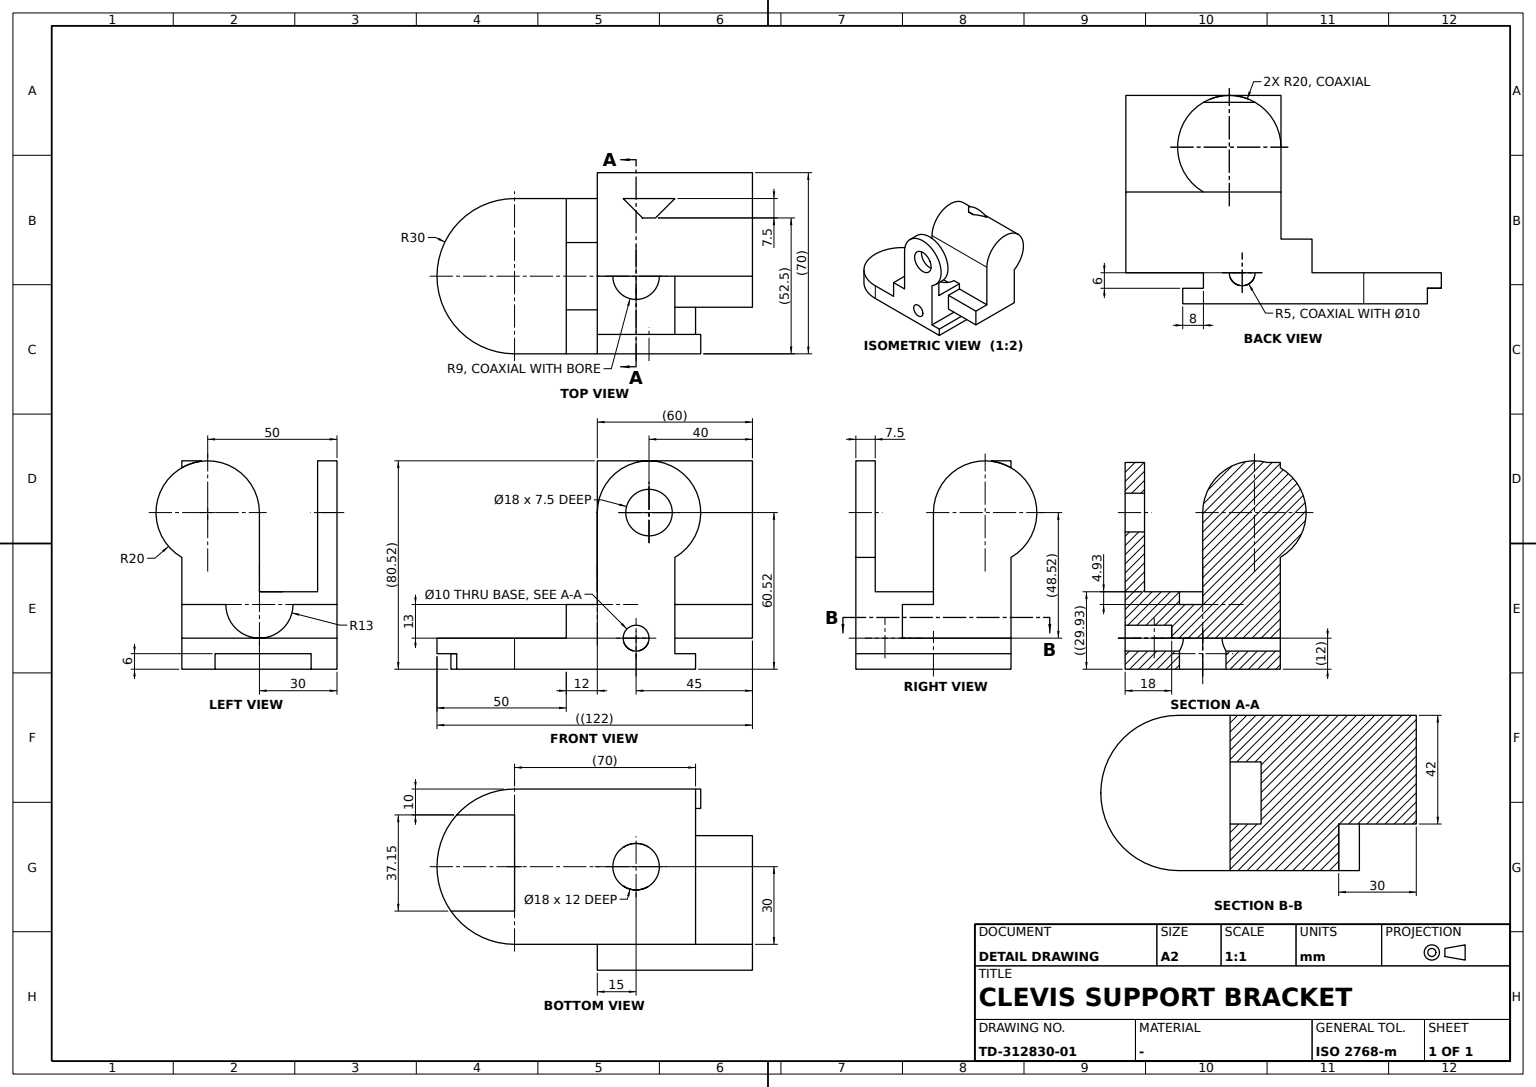
ISO-10303-21;
HEADER;
FILE_DESCRIPTION((''),'2;1');
FILE_NAME('','',(''),(''),'','','');
FILE_SCHEMA(('AUTOMOTIVE_DESIGN'));
ENDSEC;
DATA;
#1=APPLICATION_CONTEXT('');
#2=PRODUCT_CONTEXT('',#1,'mechanical');
#3=PRODUCT('','','',(#2));
#4=PRODUCT_DEFINITION_FORMATION('','',#3);
#5=PRODUCT_DEFINITION_CONTEXT('',#1,'design');
#6=PRODUCT_DEFINITION('','',#4,#5);
#7=PRODUCT_DEFINITION_SHAPE('','',#6);
#8=(LENGTH_UNIT()NAMED_UNIT(*)SI_UNIT(.MILLI.,.METRE.));
#9=(NAMED_UNIT(*)PLANE_ANGLE_UNIT()SI_UNIT($,.RADIAN.));
#10=(NAMED_UNIT(*)SI_UNIT($,.STERADIAN.)SOLID_ANGLE_UNIT());
#11=UNCERTAINTY_MEASURE_WITH_UNIT(LENGTH_MEASURE(1.E-05),#8,'distance_accuracy_value','');
#12=(GEOMETRIC_REPRESENTATION_CONTEXT(3)GLOBAL_UNCERTAINTY_ASSIGNED_CONTEXT((#11))GLOBAL_UNIT_ASSIGNED_CONTEXT((#8,#9,#10))REPRESENTATION_CONTEXT('',''));
#13=CARTESIAN_POINT('',(0.,-56.,25.));
#14=VERTEX_POINT('',#13);
#15=CARTESIAN_POINT('',(-9.,-47.,25.));
#16=VERTEX_POINT('',#15);
#17=CARTESIAN_POINT('',(0.,-47.,25.));
#18=DIRECTION('',(0.,0.,-1.));
#19=DIRECTION('',(0.,-1.,0.));
#20=AXIS2_PLACEMENT_3D('',#17,#18,#19);
#21=CIRCLE('',#20,9.);
#22=EDGE_CURVE('',#14,#16,#21,.T.);
#23=ORIENTED_EDGE('',*,*,#22,.F.);
#24=CARTESIAN_POINT('',(0.,-38.,25.));
#25=VERTEX_POINT('',#24);
#26=VECTOR('',#19,1000.);
#27=LINE('',#17,#26);
#28=EDGE_CURVE('',#25,#14,#27,.T.);
#29=ORIENTED_EDGE('',*,*,#28,.F.);
#30=EDGE_CURVE('',#16,#25,#21,.T.);
#31=ORIENTED_EDGE('',*,*,#30,.F.);
#32=EDGE_LOOP('',(#23,#29,#31));
#33=FACE_OUTER_BOUND('',#32,.T.);
#34=CARTESIAN_POINT('',(30.,-20.,25.));
#35=AXIS2_PLACEMENT_3D('',#34,#18,#19);
#36=PLANE('',#35);
#37=ADVANCED_FACE('',(#33),#36,.F.);
#38=CARTESIAN_POINT('',(-30.,0.,0.));
#39=VERTEX_POINT('',#38);
#40=CARTESIAN_POINT('',(-30.,0.,12.));
#41=VERTEX_POINT('',#40);
#42=CARTESIAN_POINT('',(-30.,0.,6.));
#43=DIRECTION('',(0.,0.,1.));
#44=VECTOR('',#43,1000.);
#45=LINE('',#42,#44);
#46=EDGE_CURVE('',#39,#41,#45,.T.);
#47=ORIENTED_EDGE('',*,*,#46,.F.);
#48=CARTESIAN_POINT('',(-30.,-20.,0.));
#49=VERTEX_POINT('',#48);
#50=CARTESIAN_POINT('',(-30.,-10.,0.));
#51=LINE('',#50,#26);
#52=EDGE_CURVE('',#39,#49,#51,.T.);
#53=ORIENTED_EDGE('',*,*,#52,.T.);
#54=CARTESIAN_POINT('',(-30.,-20.,12.));
#55=VERTEX_POINT('',#54);
#56=CARTESIAN_POINT('',(-30.,-20.,6.));
#57=LINE('',#56,#44);
#58=EDGE_CURVE('',#49,#55,#57,.T.);
#59=ORIENTED_EDGE('',*,*,#58,.T.);
#60=CARTESIAN_POINT('',(-30.,-10.,12.));
#61=LINE('',#60,#26);
#62=EDGE_CURVE('',#41,#55,#61,.T.);
#63=ORIENTED_EDGE('',*,*,#62,.F.);
#64=EDGE_LOOP('',(#47,#53,#59,#63));
#65=FACE_OUTER_BOUND('',#64,.T.);
#66=DIRECTION('',(-1.,0.,0.));
#67=AXIS2_PLACEMENT_3D('',#38,#66,#19);
#68=PLANE('',#67);
#69=ADVANCED_FACE('',(#65),#68,.T.);
#70=CARTESIAN_POINT('',(-12.,-92.,25.));
#71=VERTEX_POINT('',#70);
#72=CARTESIAN_POINT('',(0.,-92.,25.));
#73=VERTEX_POINT('',#72);
#74=CARTESIAN_POINT('',(-6.,-92.,25.));
#75=DIRECTION('',(1.,0.,0.));
#76=VECTOR('',#75,1000.);
#77=LINE('',#74,#76);
#78=EDGE_CURVE('',#71,#73,#77,.T.);
#79=ORIENTED_EDGE('',*,*,#78,.F.);
#80=CARTESIAN_POINT('',(-12.,-92.,12.));
#81=VERTEX_POINT('',#80);
#82=CARTESIAN_POINT('',(-12.,-92.,18.5));
#83=LINE('',#82,#44);
#84=EDGE_CURVE('',#81,#71,#83,.T.);
#85=ORIENTED_EDGE('',*,*,#84,.F.);
#86=CARTESIAN_POINT('',(30.,-92.,12.));
#87=VERTEX_POINT('',#86);
#88=CARTESIAN_POINT('',(9.,-92.,12.));
#89=VECTOR('',#66,1000.);
#90=LINE('',#88,#89);
#91=EDGE_CURVE('',#87,#81,#90,.T.);
#92=ORIENTED_EDGE('',*,*,#91,.F.);
#93=CARTESIAN_POINT('',(30.,-92.,43.201274));
#94=VERTEX_POINT('',#93);
#95=CARTESIAN_POINT('',(30.,-92.,27.600637));
#96=VECTOR('',#18,1000.);
#97=LINE('',#95,#96);
#98=EDGE_CURVE('',#94,#87,#97,.T.);
#99=ORIENTED_EDGE('',*,*,#98,.F.);
#100=CARTESIAN_POINT('',(0.,-92.,60.521782));
#101=VERTEX_POINT('',#100);
#102=CARTESIAN_POINT('',(20.,-92.,60.521782));
#103=DIRECTION('',(0.,1.,0.));
#104=AXIS2_PLACEMENT_3D('',#102,#103,#66);
#105=CIRCLE('',#104,20.);
#106=EDGE_CURVE('',#101,#94,#105,.T.);
#107=ORIENTED_EDGE('',*,*,#106,.F.);
#108=CARTESIAN_POINT('',(0.,-92.,42.760891));
#109=LINE('',#108,#44);
#110=EDGE_CURVE('',#73,#101,#109,.T.);
#111=ORIENTED_EDGE('',*,*,#110,.F.);
#112=EDGE_LOOP('',(#79,#85,#92,#99,#107,#111));
#113=FACE_OUTER_BOUND('',#112,.T.);
#114=CARTESIAN_POINT('',(0.,-92.,0.));
#115=AXIS2_PLACEMENT_3D('',#114,#103,#66);
#116=PLANE('',#115);
#117=ADVANCED_FACE('',(#113),#116,.F.);
#118=CARTESIAN_POINT('',(-9.,-47.,29.92601));
#119=VERTEX_POINT('',#118);
#120=CARTESIAN_POINT('',(-9.,-47.,14.303005));
#121=LINE('',#120,#96);
#122=EDGE_CURVE('',#119,#16,#121,.T.);
#123=ORIENTED_EDGE('',*,*,#122,.F.);
#124=CARTESIAN_POINT('',(0.,-56.,29.92601));
#125=VERTEX_POINT('',#124);
#126=CARTESIAN_POINT('',(0.,-47.,29.92601));
#127=AXIS2_PLACEMENT_3D('',#126,#18,#75);
#128=CIRCLE('',#127,9.);
#129=EDGE_CURVE('',#125,#119,#128,.T.);
#130=ORIENTED_EDGE('',*,*,#129,.F.);
#131=CARTESIAN_POINT('',(0.,-56.,27.463005));
#132=LINE('',#131,#96);
#133=EDGE_CURVE('',#125,#14,#132,.T.);
#134=ORIENTED_EDGE('',*,*,#133,.T.);
#135=ORIENTED_EDGE('',*,*,#22,.T.);
#136=EDGE_LOOP('',(#123,#130,#134,#135));
#137=FACE_OUTER_BOUND('',#136,.T.);
#138=CARTESIAN_POINT('',(0.,-47.,14.303005));
#139=AXIS2_PLACEMENT_3D('',#138,#43,#75);
#140=CYLINDRICAL_SURFACE('',#139,9.);
#141=ADVANCED_FACE('',(#137),#140,.F.);
#142=CARTESIAN_POINT('',(30.,-20.,12.));
#143=VERTEX_POINT('',#142);
#144=CARTESIAN_POINT('',(0.,-20.,12.));
#145=VERTEX_POINT('',#144);
#146=CARTESIAN_POINT('',(15.,-20.,12.));
#147=LINE('',#146,#89);
#148=EDGE_CURVE('',#143,#145,#147,.T.);
#149=ORIENTED_EDGE('',*,*,#148,.T.);
#150=CARTESIAN_POINT('',(13.,-20.,25.));
#151=VERTEX_POINT('',#150);
#152=CARTESIAN_POINT('',(0.,-20.,25.));
#153=AXIS2_PLACEMENT_3D('',#152,#103,#66);
#154=CIRCLE('',#153,13.);
#155=EDGE_CURVE('',#151,#145,#154,.T.);
#156=ORIENTED_EDGE('',*,*,#155,.F.);
#157=VERTEX_POINT('',#34);
#158=CARTESIAN_POINT('',(21.5,-20.,25.));
#159=LINE('',#158,#89);
#160=EDGE_CURVE('',#157,#151,#159,.T.);
#161=ORIENTED_EDGE('',*,*,#160,.F.);
#162=CARTESIAN_POINT('',(30.,-20.,18.5));
#163=LINE('',#162,#44);
#164=EDGE_CURVE('',#143,#157,#163,.T.);
#165=ORIENTED_EDGE('',*,*,#164,.F.);
#166=EDGE_LOOP('',(#149,#156,#161,#165));
#167=FACE_OUTER_BOUND('',#166,.T.);
#168=AXIS2_PLACEMENT_3D('',#142,#19,#43);
#169=PLANE('',#168);
#170=ADVANCED_FACE('',(#167),#169,.F.);
#171=CARTESIAN_POINT('',(30.,-70.,6.));
#172=VERTEX_POINT('',#171);
#173=CARTESIAN_POINT('',(30.,-62.,6.));
#174=VERTEX_POINT('',#173);
#175=CARTESIAN_POINT('',(30.,-66.,6.));
#176=VECTOR('',#103,1000.);
#177=LINE('',#175,#176);
#178=EDGE_CURVE('',#172,#174,#177,.T.);
#179=ORIENTED_EDGE('',*,*,#178,.T.);
#180=CARTESIAN_POINT('',(-30.,-62.,6.));
#181=VERTEX_POINT('',#180);
#182=CARTESIAN_POINT('',(0.,-62.,6.));
#183=LINE('',#182,#89);
#184=EDGE_CURVE('',#174,#181,#183,.T.);
#185=ORIENTED_EDGE('',*,*,#184,.T.);
#186=CARTESIAN_POINT('',(-30.,-70.,6.));
#187=VERTEX_POINT('',#186);
#188=CARTESIAN_POINT('',(-30.,-66.,6.));
#189=LINE('',#188,#176);
#190=EDGE_CURVE('',#187,#181,#189,.T.);
#191=ORIENTED_EDGE('',*,*,#190,.F.);
#192=CARTESIAN_POINT('',(0.,-70.,6.));
#193=LINE('',#192,#89);
#194=EDGE_CURVE('',#172,#187,#193,.T.);
#195=ORIENTED_EDGE('',*,*,#194,.F.);
#196=EDGE_LOOP('',(#179,#185,#191,#195));
#197=FACE_OUTER_BOUND('',#196,.T.);
#198=AXIS2_PLACEMENT_3D('',#173,#18,#19);
#199=PLANE('',#198);
#200=ADVANCED_FACE('',(#197),#199,.F.);
#201=CARTESIAN_POINT('',(0.,-38.,29.92601));
#202=VERTEX_POINT('',#201);
#203=EDGE_CURVE('',#119,#202,#128,.T.);
#204=ORIENTED_EDGE('',*,*,#203,.F.);
#205=ORIENTED_EDGE('',*,*,#122,.T.);
#206=ORIENTED_EDGE('',*,*,#30,.T.);
#207=CARTESIAN_POINT('',(0.,-38.,27.463005));
#208=LINE('',#207,#96);
#209=EDGE_CURVE('',#202,#25,#208,.T.);
#210=ORIENTED_EDGE('',*,*,#209,.F.);
#211=EDGE_LOOP('',(#204,#205,#206,#210));
#212=FACE_OUTER_BOUND('',#211,.T.);
#213=ADVANCED_FACE('',(#212),#140,.F.);
#214=CARTESIAN_POINT('',(30.,-70.,0.));
#215=VERTEX_POINT('',#214);
#216=CARTESIAN_POINT('',(30.,-70.,3.));
#217=LINE('',#216,#44);
#218=EDGE_CURVE('',#215,#172,#217,.T.);
#219=ORIENTED_EDGE('',*,*,#218,.T.);
#220=ORIENTED_EDGE('',*,*,#194,.T.);
#221=CARTESIAN_POINT('',(-30.,-70.,0.));
#222=VERTEX_POINT('',#221);
#223=CARTESIAN_POINT('',(-30.,-70.,3.));
#224=LINE('',#223,#44);
#225=EDGE_CURVE('',#222,#187,#224,.T.);
#226=ORIENTED_EDGE('',*,*,#225,.F.);
#227=CARTESIAN_POINT('',(0.,-70.,0.));
#228=LINE('',#227,#76);
#229=EDGE_CURVE('',#222,#215,#228,.T.);
#230=ORIENTED_EDGE('',*,*,#229,.T.);
#231=EDGE_LOOP('',(#219,#220,#226,#230));
#232=FACE_OUTER_BOUND('',#231,.T.);
#233=AXIS2_PLACEMENT_3D('',#221,#19,#75);
#234=PLANE('',#233);
#235=ADVANCED_FACE('',(#232),#234,.T.);
#236=CARTESIAN_POINT('',(-20.,0.,6.));
#237=VERTEX_POINT('',#236);
#238=CARTESIAN_POINT('',(17.153702,0.,6.));
#239=VERTEX_POINT('',#238);
#240=CARTESIAN_POINT('',(-1.423149,0.,6.));
#241=LINE('',#240,#76);
#242=EDGE_CURVE('',#237,#239,#241,.T.);
#243=ORIENTED_EDGE('',*,*,#242,.F.);
#244=CARTESIAN_POINT('',(-20.,22.36068,6.));
#245=VERTEX_POINT('',#244);
#246=CARTESIAN_POINT('',(-20.,11.18034,6.));
#247=LINE('',#246,#176);
#248=EDGE_CURVE('',#237,#245,#247,.T.);
#249=ORIENTED_EDGE('',*,*,#248,.T.);
#250=CARTESIAN_POINT('',(0.,30.,6.));
#251=VERTEX_POINT('',#250);
#252=CARTESIAN_POINT('',(0.,0.,6.));
#253=AXIS2_PLACEMENT_3D('',#252,#18,#19);
#254=CIRCLE('',#253,30.);
#255=EDGE_CURVE('',#245,#251,#254,.T.);
#256=ORIENTED_EDGE('',*,*,#255,.T.);
#257=CARTESIAN_POINT('',(17.153702,24.611999,6.));
#258=VERTEX_POINT('',#257);
#259=EDGE_CURVE('',#251,#258,#254,.T.);
#260=ORIENTED_EDGE('',*,*,#259,.T.);
#261=CARTESIAN_POINT('',(17.153702,12.306,6.));
#262=LINE('',#261,#176);
#263=EDGE_CURVE('',#239,#258,#262,.T.);
#264=ORIENTED_EDGE('',*,*,#263,.F.);
#265=EDGE_LOOP('',(#243,#249,#256,#260,#264));
#266=FACE_OUTER_BOUND('',#265,.T.);
#267=ADVANCED_FACE('',(#266),#199,.T.);
#268=CARTESIAN_POINT('',(-9.,-47.,7.));
#269=VERTEX_POINT('',#268);
#270=CARTESIAN_POINT('',(-9.,-47.,0.));
#271=VERTEX_POINT('',#270);
#272=EDGE_CURVE('',#269,#271,#121,.T.);
#273=ORIENTED_EDGE('',*,*,#272,.T.);
#274=CARTESIAN_POINT('',(9.,-47.,0.));
#275=VERTEX_POINT('',#274);
#276=CARTESIAN_POINT('',(0.,-47.,0.));
#277=AXIS2_PLACEMENT_3D('',#276,#43,#103);
#278=CIRCLE('',#277,9.);
#279=EDGE_CURVE('',#275,#271,#278,.T.);
#280=ORIENTED_EDGE('',*,*,#279,.F.);
#281=CARTESIAN_POINT('',(9.,-47.,7.));
#282=VERTEX_POINT('',#281);
#283=CARTESIAN_POINT('',(9.,-47.,14.303005));
#284=LINE('',#283,#96);
#285=EDGE_CURVE('',#282,#275,#284,.T.);
#286=ORIENTED_EDGE('',*,*,#285,.F.);
#287=CARTESIAN_POINT('',(7.483315,-42.,12.));
#288=VERTEX_POINT('',#287);
#289=CARTESIAN_POINT('',(7.483315,-42.,11.685205));
#290=CARTESIAN_POINT('',(7.499868,-42.024774,11.370411));
#291=CARTESIAN_POINT('',(7.532989,-42.074315,11.059602));
#292=CARTESIAN_POINT('',(7.610371,-42.193209,10.565487));
#293=CARTESIAN_POINT('',(7.718669,-42.370486,10.096475));
#294=CARTESIAN_POINT('',(7.764337,-42.447141,9.919954));
#295=CARTESIAN_POINT('',(7.887461,-42.660396,9.486778));
#296=CARTESIAN_POINT('',(8.026315,-42.92214,9.085241));
#297=CARTESIAN_POINT('',(8.113397,-43.096714,8.855373));
#298=CARTESIAN_POINT('',(8.289483,-43.477417,8.422429));
#299=CARTESIAN_POINT('',(8.460682,-43.917285,8.04753));
#300=CARTESIAN_POINT('',(8.542878,-44.151027,7.875708));
#301=CARTESIAN_POINT('',(8.696396,-44.643878,7.565776));
#302=CARTESIAN_POINT('',(8.821262,-45.182747,7.327965));
#303=CARTESIAN_POINT('',(8.87472,-45.462214,7.228426));
#304=CARTESIAN_POINT('',(8.945181,-45.934634,7.098983));
#305=CARTESIAN_POINT('',(8.984478,-46.421778,7.027938));
#306=CARTESIAN_POINT('',(8.994826,-46.613989,7.009313));
#307=CARTESIAN_POINT('',(9.,-46.806994,7.));
#308=B_SPLINE_CURVE_WITH_KNOTS('',5,(#287,#289,#290,#291,#292,#293,#294,#295,#296,#297,#298,#299,#300,#301,#302,#303,#304,#305,#306,#307,#281),.UNSPECIFIED.,.F.,.F.,(6,3,3,3,3,3,6),(0.,2.225934193,3.62206107,5.745254465,7.86844786,9.990789164,11.35554502),.UNSPECIFIED.);
#309=EDGE_CURVE('',#288,#282,#308,.T.);
#310=ORIENTED_EDGE('',*,*,#309,.F.);
#311=CARTESIAN_POINT('',(-7.483315,-42.,12.));
#312=VERTEX_POINT('',#311);
#313=CARTESIAN_POINT('',(0.,-47.,12.));
#314=AXIS2_PLACEMENT_3D('',#313,#43,#103);
#315=CIRCLE('',#314,9.);
#316=EDGE_CURVE('',#288,#312,#315,.T.);
#317=ORIENTED_EDGE('',*,*,#316,.T.);
#318=CARTESIAN_POINT('',(-7.483315,-42.,11.685205));
#319=CARTESIAN_POINT('',(-7.499868,-42.024774,11.370411));
#320=CARTESIAN_POINT('',(-7.532989,-42.074315,11.059602));
#321=CARTESIAN_POINT('',(-7.610371,-42.193209,10.565487));
#322=CARTESIAN_POINT('',(-7.718669,-42.370486,10.096475));
#323=CARTESIAN_POINT('',(-7.764337,-42.447141,9.919954));
#324=CARTESIAN_POINT('',(-7.887461,-42.660396,9.486778));
#325=CARTESIAN_POINT('',(-8.026315,-42.92214,9.085241));
#326=CARTESIAN_POINT('',(-8.113397,-43.096714,8.855373));
#327=CARTESIAN_POINT('',(-8.289483,-43.477417,8.422429));
#328=CARTESIAN_POINT('',(-8.460682,-43.917285,8.04753));
#329=CARTESIAN_POINT('',(-8.542878,-44.151027,7.875708));
#330=CARTESIAN_POINT('',(-8.696396,-44.643878,7.565776));
#331=CARTESIAN_POINT('',(-8.821262,-45.182747,7.327965));
#332=CARTESIAN_POINT('',(-8.87472,-45.462214,7.228426));
#333=CARTESIAN_POINT('',(-8.945181,-45.934634,7.098983));
#334=CARTESIAN_POINT('',(-8.984478,-46.421778,7.027938));
#335=CARTESIAN_POINT('',(-8.994826,-46.613989,7.009313));
#336=CARTESIAN_POINT('',(-9.,-46.806994,7.));
#337=B_SPLINE_CURVE_WITH_KNOTS('',5,(#311,#318,#319,#320,#321,#322,#323,#324,#325,#326,#327,#328,#329,#330,#331,#332,#333,#334,#335,#336,#268),.UNSPECIFIED.,.F.,.F.,(6,3,3,3,3,3,6),(0.,2.225934193,3.62206107,5.745254465,7.868447861,9.990789164,11.35554502),.UNSPECIFIED.);
#338=EDGE_CURVE('',#312,#269,#337,.T.);
#339=ORIENTED_EDGE('',*,*,#338,.T.);
#340=EDGE_LOOP('',(#273,#280,#286,#310,#317,#339));
#341=FACE_OUTER_BOUND('',#340,.T.);
#342=ADVANCED_FACE('',(#341),#140,.F.);
#343=CARTESIAN_POINT('',(13.,-32.,25.));
#344=VERTEX_POINT('',#343);
#345=CARTESIAN_POINT('',(-13.,-32.,25.));
#346=VERTEX_POINT('',#345);
#347=CARTESIAN_POINT('',(0.,-32.,25.));
#348=AXIS2_PLACEMENT_3D('',#347,#103,#66);
#349=CIRCLE('',#348,13.);
#350=EDGE_CURVE('',#344,#346,#349,.T.);
#351=ORIENTED_EDGE('',*,*,#350,.T.);
#352=CARTESIAN_POINT('',(-30.,-32.,25.));
#353=VERTEX_POINT('',#352);
#354=CARTESIAN_POINT('',(-21.5,-32.,25.));
#355=LINE('',#354,#89);
#356=EDGE_CURVE('',#346,#353,#355,.T.);
#357=ORIENTED_EDGE('',*,*,#356,.T.);
#358=CARTESIAN_POINT('',(-30.,-32.,60.521782));
#359=VERTEX_POINT('',#358);
#360=CARTESIAN_POINT('',(-30.,-32.,42.760891));
#361=LINE('',#360,#44);
#362=EDGE_CURVE('',#353,#359,#361,.T.);
#363=ORIENTED_EDGE('',*,*,#362,.T.);
#364=CARTESIAN_POINT('',(-22.5,-32.,60.521782));
#365=VERTEX_POINT('',#364);
#366=CARTESIAN_POINT('',(-26.25,-32.,60.521782));
#367=LINE('',#366,#89);
#368=EDGE_CURVE('',#365,#359,#367,.T.);
#369=ORIENTED_EDGE('',*,*,#368,.F.);
#370=CARTESIAN_POINT('',(-22.5,-32.,29.92601));
#371=VERTEX_POINT('',#370);
#372=CARTESIAN_POINT('',(-22.5,-32.,45.223896));
#373=LINE('',#372,#44);
#374=EDGE_CURVE('',#371,#365,#373,.T.);
#375=ORIENTED_EDGE('',*,*,#374,.F.);
#376=CARTESIAN_POINT('',(0.,-32.,29.92601));
#377=VERTEX_POINT('',#376);
#378=CARTESIAN_POINT('',(-11.25,-32.,29.92601));
#379=LINE('',#378,#89);
#380=EDGE_CURVE('',#377,#371,#379,.T.);
#381=ORIENTED_EDGE('',*,*,#380,.F.);
#382=CARTESIAN_POINT('',(0.,-32.,60.521782));
#383=VERTEX_POINT('',#382);
#384=CARTESIAN_POINT('',(0.,-32.,45.223896));
#385=LINE('',#384,#44);
#386=EDGE_CURVE('',#377,#383,#385,.T.);
#387=ORIENTED_EDGE('',*,*,#386,.T.);
#388=CARTESIAN_POINT('',(30.,-32.,43.201274));
#389=VERTEX_POINT('',#388);
#390=CARTESIAN_POINT('',(20.,-32.,60.521782));
#391=AXIS2_PLACEMENT_3D('',#390,#103,#66);
#392=CIRCLE('',#391,20.);
#393=EDGE_CURVE('',#383,#389,#392,.T.);
#394=ORIENTED_EDGE('',*,*,#393,.T.);
#395=CARTESIAN_POINT('',(30.,-32.,25.));
#396=VERTEX_POINT('',#395);
#397=CARTESIAN_POINT('',(30.,-32.,34.100637));
#398=LINE('',#397,#96);
#399=EDGE_CURVE('',#389,#396,#398,.T.);
#400=ORIENTED_EDGE('',*,*,#399,.T.);
#401=CARTESIAN_POINT('',(21.5,-32.,25.));
#402=LINE('',#401,#89);
#403=EDGE_CURVE('',#396,#344,#402,.T.);
#404=ORIENTED_EDGE('',*,*,#403,.T.);
#405=EDGE_LOOP('',(#351,#357,#363,#369,#375,#381,#387,#394,#400,#404));
#406=FACE_OUTER_BOUND('',#405,.T.);
#407=AXIS2_PLACEMENT_3D('',#395,#19,#43);
#408=PLANE('',#407);
#409=ADVANCED_FACE('',(#406),#408,.F.);
#410=ORIENTED_EDGE('',*,*,#368,.T.);
#411=CARTESIAN_POINT('',(-30.,-62.,43.201274));
#412=VERTEX_POINT('',#411);
#413=CARTESIAN_POINT('',(-30.,-52.,60.521782));
#414=AXIS2_PLACEMENT_3D('',#413,#75,#103);
#415=CIRCLE('',#414,20.);
#416=EDGE_CURVE('',#359,#412,#415,.T.);
#417=ORIENTED_EDGE('',*,*,#416,.T.);
#418=CARTESIAN_POINT('',(-22.5,-62.,43.201274));
#419=VERTEX_POINT('',#418);
#420=CARTESIAN_POINT('',(0.,-62.,43.201274));
#421=LINE('',#420,#89);
#422=EDGE_CURVE('',#419,#412,#421,.T.);
#423=ORIENTED_EDGE('',*,*,#422,.F.);
#424=CARTESIAN_POINT('',(-22.5,-52.,60.521782));
#425=AXIS2_PLACEMENT_3D('',#424,#75,#43);
#426=CIRCLE('',#425,20.);
#427=EDGE_CURVE('',#365,#419,#426,.T.);
#428=ORIENTED_EDGE('',*,*,#427,.F.);
#429=EDGE_LOOP('',(#410,#417,#423,#428));
#430=FACE_OUTER_BOUND('',#429,.T.);
#431=CARTESIAN_POINT('',(0.,-52.,60.521782));
#432=AXIS2_PLACEMENT_3D('',#431,#66,#103);
#433=CYLINDRICAL_SURFACE('',#432,20.);
#434=ADVANCED_FACE('',(#430),#433,.T.);
#435=CARTESIAN_POINT('',(17.153702,0.,0.));
#436=VERTEX_POINT('',#435);
#437=CARTESIAN_POINT('',(17.153702,0.,3.));
#438=LINE('',#437,#96);
#439=EDGE_CURVE('',#239,#436,#438,.T.);
#440=ORIENTED_EDGE('',*,*,#439,.T.);
#441=CARTESIAN_POINT('',(-20.,0.,0.));
#442=VERTEX_POINT('',#441);
#443=CARTESIAN_POINT('',(-1.423149,0.,0.));
#444=LINE('',#443,#89);
#445=EDGE_CURVE('',#436,#442,#444,.T.);
#446=ORIENTED_EDGE('',*,*,#445,.T.);
#447=CARTESIAN_POINT('',(-20.,0.,3.));
#448=LINE('',#447,#44);
#449=EDGE_CURVE('',#442,#237,#448,.T.);
#450=ORIENTED_EDGE('',*,*,#449,.T.);
#451=ORIENTED_EDGE('',*,*,#242,.T.);
#452=EDGE_LOOP('',(#440,#446,#450,#451));
#453=FACE_OUTER_BOUND('',#452,.T.);
#454=CARTESIAN_POINT('',(0.,0.,0.));
#455=AXIS2_PLACEMENT_3D('',#454,#103,#66);
#456=PLANE('',#455);
#457=ADVANCED_FACE('',(#453),#456,.T.);
#458=CARTESIAN_POINT('',(17.153702,24.611999,0.));
#459=VERTEX_POINT('',#458);
#460=CARTESIAN_POINT('',(17.153702,12.306,0.));
#461=LINE('',#460,#176);
#462=EDGE_CURVE('',#436,#459,#461,.T.);
#463=ORIENTED_EDGE('',*,*,#462,.F.);
#464=ORIENTED_EDGE('',*,*,#439,.F.);
#465=ORIENTED_EDGE('',*,*,#263,.T.);
#466=CARTESIAN_POINT('',(17.153702,24.611999,3.));
#467=LINE('',#466,#96);
#468=EDGE_CURVE('',#258,#459,#467,.T.);
#469=ORIENTED_EDGE('',*,*,#468,.T.);
#470=EDGE_LOOP('',(#463,#464,#465,#469));
#471=FACE_OUTER_BOUND('',#470,.T.);
#472=AXIS2_PLACEMENT_3D('',#238,#75,#18);
#473=PLANE('',#472);
#474=ADVANCED_FACE('',(#471),#473,.F.);
#475=CARTESIAN_POINT('',(13.,-26.,25.));
#476=LINE('',#475,#26);
#477=EDGE_CURVE('',#151,#344,#476,.T.);
#478=ORIENTED_EDGE('',*,*,#477,.F.);
#479=ORIENTED_EDGE('',*,*,#155,.T.);
#480=CARTESIAN_POINT('',(-13.,-20.,25.));
#481=VERTEX_POINT('',#480);
#482=EDGE_CURVE('',#145,#481,#154,.T.);
#483=ORIENTED_EDGE('',*,*,#482,.T.);
#484=CARTESIAN_POINT('',(-13.,-26.,25.));
#485=LINE('',#484,#26);
#486=EDGE_CURVE('',#481,#346,#485,.T.);
#487=ORIENTED_EDGE('',*,*,#486,.T.);
#488=ORIENTED_EDGE('',*,*,#350,.F.);
#489=EDGE_LOOP('',(#478,#479,#483,#487,#488));
#490=FACE_OUTER_BOUND('',#489,.T.);
#491=CARTESIAN_POINT('',(0.,-26.,25.));
#492=AXIS2_PLACEMENT_3D('',#491,#19,#66);
#493=CYLINDRICAL_SURFACE('',#492,13.);
#494=ADVANCED_FACE('',(#490),#493,.F.);
#495=CARTESIAN_POINT('',(-15.,-20.,12.));
#496=LINE('',#495,#89);
#497=EDGE_CURVE('',#145,#55,#496,.T.);
#498=ORIENTED_EDGE('',*,*,#497,.F.);
#499=ORIENTED_EDGE('',*,*,#148,.F.);
#500=CARTESIAN_POINT('',(30.,0.,12.));
#501=VERTEX_POINT('',#500);
#502=CARTESIAN_POINT('',(30.,-10.,12.));
#503=LINE('',#502,#176);
#504=EDGE_CURVE('',#143,#501,#503,.T.);
#505=ORIENTED_EDGE('',*,*,#504,.T.);
#506=CARTESIAN_POINT('',(0.,30.,12.));
#507=VERTEX_POINT('',#506);
#508=CARTESIAN_POINT('',(0.,0.,12.));
#509=AXIS2_PLACEMENT_3D('',#508,#43,#103);
#510=CIRCLE('',#509,30.);
#511=EDGE_CURVE('',#501,#507,#510,.T.);
#512=ORIENTED_EDGE('',*,*,#511,.T.);
#513=EDGE_CURVE('',#507,#41,#510,.T.);
#514=ORIENTED_EDGE('',*,*,#513,.T.);
#515=ORIENTED_EDGE('',*,*,#62,.T.);
#516=EDGE_LOOP('',(#498,#499,#505,#512,#514,#515));
#517=FACE_OUTER_BOUND('',#516,.T.);
#518=PLANE('',#509);
#519=ADVANCED_FACE('',(#517),#518,.T.);
#520=ORIENTED_EDGE('',*,*,#91,.T.);
#521=CARTESIAN_POINT('',(-12.,-62.,12.));
#522=VERTEX_POINT('',#521);
#523=CARTESIAN_POINT('',(-12.,-77.,12.));
#524=LINE('',#523,#26);
#525=EDGE_CURVE('',#522,#81,#524,.T.);
#526=ORIENTED_EDGE('',*,*,#525,.F.);
#527=CARTESIAN_POINT('',(30.,-62.,12.));
#528=VERTEX_POINT('',#527);
#529=CARTESIAN_POINT('',(9.,-62.,12.));
#530=LINE('',#529,#89);
#531=EDGE_CURVE('',#528,#522,#530,.T.);
#532=ORIENTED_EDGE('',*,*,#531,.F.);
#533=CARTESIAN_POINT('',(30.,-77.,12.));
#534=LINE('',#533,#26);
#535=EDGE_CURVE('',#528,#87,#534,.T.);
#536=ORIENTED_EDGE('',*,*,#535,.T.);
#537=EDGE_LOOP('',(#520,#526,#532,#536));
#538=FACE_OUTER_BOUND('',#537,.T.);
#539=ADVANCED_FACE('',(#538),#518,.F.);
#540=CARTESIAN_POINT('',(-12.,-52.,12.));
#541=VERTEX_POINT('',#540);
#542=CARTESIAN_POINT('',(-30.,-52.,12.));
#543=VERTEX_POINT('',#542);
#544=CARTESIAN_POINT('',(-0.66,-52.,12.));
#545=LINE('',#544,#89);
#546=EDGE_CURVE('',#541,#543,#545,.T.);
#547=ORIENTED_EDGE('',*,*,#546,.T.);
#548=CARTESIAN_POINT('',(-30.,-42.,12.));
#549=VERTEX_POINT('',#548);
#550=CARTESIAN_POINT('',(-30.,-47.,12.));
#551=AXIS2_PLACEMENT_3D('',#550,#66,#19);
#552=CIRCLE('',#551,5.);
#553=EDGE_CURVE('',#543,#549,#552,.T.);
#554=ORIENTED_EDGE('',*,*,#553,.T.);
#555=CARTESIAN_POINT('',(-12.,-42.,12.));
#556=VERTEX_POINT('',#555);
#557=CARTESIAN_POINT('',(-0.66,-42.,12.));
#558=LINE('',#557,#89);
#559=EDGE_CURVE('',#556,#549,#558,.T.);
#560=ORIENTED_EDGE('',*,*,#559,.F.);
#561=CARTESIAN_POINT('',(-12.,-47.,12.));
#562=AXIS2_PLACEMENT_3D('',#561,#75,#43);
#563=CIRCLE('',#562,5.);
#564=EDGE_CURVE('',#556,#541,#563,.T.);
#565=ORIENTED_EDGE('',*,*,#564,.T.);
#566=EDGE_LOOP('',(#547,#554,#560,#565));
#567=FACE_OUTER_BOUND('',#566,.T.);
#568=CARTESIAN_POINT('',(-0.66,-47.,12.));
#569=AXIS2_PLACEMENT_3D('',#568,#66,#103);
#570=CYLINDRICAL_SURFACE('',#569,5.);
#571=ADVANCED_FACE('',(#567),#570,.F.);
#572=EDGE_CURVE('',#549,#543,#552,.T.);
#573=ORIENTED_EDGE('',*,*,#572,.F.);
#574=ORIENTED_EDGE('',*,*,#553,.F.);
#575=EDGE_LOOP('',(#573,#574));
#576=FACE_BOUND('',#575,.T.);
#577=CARTESIAN_POINT('',(-30.,-43.,60.521782));
#578=VERTEX_POINT('',#577);
#579=CARTESIAN_POINT('',(-30.,-44.101757,56.206952));
#580=VERTEX_POINT('',#579);
#581=AXIS2_PLACEMENT_3D('',#413,#66,#19);
#582=CIRCLE('',#581,9.);
#583=EDGE_CURVE('',#578,#580,#582,.T.);
#584=ORIENTED_EDGE('',*,*,#583,.F.);
#585=CARTESIAN_POINT('',(-30.,-59.898243,64.836612));
#586=VERTEX_POINT('',#585);
#587=EDGE_CURVE('',#586,#578,#582,.T.);
#588=ORIENTED_EDGE('',*,*,#587,.F.);
#589=EDGE_CURVE('',#580,#586,#582,.T.);
#590=ORIENTED_EDGE('',*,*,#589,.F.);
#591=EDGE_LOOP('',(#584,#588,#590));
#592=FACE_BOUND('',#591,.T.);
#593=CARTESIAN_POINT('',(-30.,-45.,0.));
#594=LINE('',#593,#26);
#595=EDGE_CURVE('',#49,#222,#594,.T.);
#596=ORIENTED_EDGE('',*,*,#595,.T.);
#597=ORIENTED_EDGE('',*,*,#225,.T.);
#598=ORIENTED_EDGE('',*,*,#190,.T.);
#599=CARTESIAN_POINT('',(-30.,-62.,24.600637));
#600=LINE('',#599,#96);
#601=EDGE_CURVE('',#412,#181,#600,.T.);
#602=ORIENTED_EDGE('',*,*,#601,.F.);
#603=ORIENTED_EDGE('',*,*,#416,.F.);
#604=ORIENTED_EDGE('',*,*,#362,.F.);
#605=CARTESIAN_POINT('',(-30.,-20.,25.));
#606=VERTEX_POINT('',#605);
#607=CARTESIAN_POINT('',(-30.,-26.,25.));
#608=LINE('',#607,#26);
#609=EDGE_CURVE('',#606,#353,#608,.T.);
#610=ORIENTED_EDGE('',*,*,#609,.F.);
#611=CARTESIAN_POINT('',(-30.,-20.,18.5));
#612=LINE('',#611,#44);
#613=EDGE_CURVE('',#55,#606,#612,.T.);
#614=ORIENTED_EDGE('',*,*,#613,.F.);
#615=ORIENTED_EDGE('',*,*,#58,.F.);
#616=EDGE_LOOP('',(#596,#597,#598,#602,#603,#604,#610,#614,#615));
#617=FACE_OUTER_BOUND('',#616,.T.);
#618=ADVANCED_FACE('',(#576,#592,#617),#68,.T.);
#619=ORIENTED_EDGE('',*,*,#84,.T.);
#620=CARTESIAN_POINT('',(-12.,-62.,25.));
#621=VERTEX_POINT('',#620);
#622=CARTESIAN_POINT('',(-12.,-77.,25.));
#623=LINE('',#622,#26);
#624=EDGE_CURVE('',#621,#71,#623,.T.);
#625=ORIENTED_EDGE('',*,*,#624,.F.);
#626=CARTESIAN_POINT('',(-12.,-62.,18.5));
#627=LINE('',#626,#44);
#628=EDGE_CURVE('',#522,#621,#627,.T.);
#629=ORIENTED_EDGE('',*,*,#628,.F.);
#630=ORIENTED_EDGE('',*,*,#525,.T.);
#631=EDGE_LOOP('',(#619,#625,#629,#630));
#632=FACE_OUTER_BOUND('',#631,.T.);
#633=CARTESIAN_POINT('',(-12.,-32.,12.));
#634=AXIS2_PLACEMENT_3D('',#633,#75,#43);
#635=PLANE('',#634);
#636=ADVANCED_FACE('',(#632),#635,.F.);
#637=CARTESIAN_POINT('',(30.,-62.,77.84229));
#638=VERTEX_POINT('',#637);
#639=CARTESIAN_POINT('',(30.,-42.,77.84229));
#640=VERTEX_POINT('',#639);
#641=CARTESIAN_POINT('',(30.,-52.,77.84229));
#642=LINE('',#641,#176);
#643=EDGE_CURVE('',#638,#640,#642,.T.);
#644=ORIENTED_EDGE('',*,*,#643,.T.);
#645=CARTESIAN_POINT('',(30.,-52.,60.521782));
#646=AXIS2_PLACEMENT_3D('',#645,#75,#103);
#647=CIRCLE('',#646,20.);
#648=EDGE_CURVE('',#640,#638,#647,.T.);
#649=ORIENTED_EDGE('',*,*,#648,.T.);
#650=EDGE_LOOP('',(#644,#649));
#651=FACE_OUTER_BOUND('',#650,.T.);
#652=CARTESIAN_POINT('',(30.,-20.,0.));
#653=AXIS2_PLACEMENT_3D('',#652,#66,#19);
#654=PLANE('',#653);
#655=ADVANCED_FACE('',(#651),#654,.F.);
#656=ORIENTED_EDGE('',*,*,#564,.F.);
#657=LINE('',#561,#26);
#658=EDGE_CURVE('',#556,#541,#657,.T.);
#659=ORIENTED_EDGE('',*,*,#658,.T.);
#660=EDGE_LOOP('',(#656,#659));
#661=FACE_OUTER_BOUND('',#660,.T.);
#662=ADVANCED_FACE('',(#661),#635,.F.);
#663=CARTESIAN_POINT('',(30.,-52.,12.));
#664=VERTEX_POINT('',#663);
#665=CARTESIAN_POINT('',(7.483315,-52.,12.));
#666=VERTEX_POINT('',#665);
#667=EDGE_CURVE('',#664,#666,#545,.T.);
#668=ORIENTED_EDGE('',*,*,#667,.F.);
#669=CARTESIAN_POINT('',(30.,-42.,12.));
#670=VERTEX_POINT('',#669);
#671=CARTESIAN_POINT('',(30.,-47.,12.));
#672=AXIS2_PLACEMENT_3D('',#671,#75,#103);
#673=CIRCLE('',#672,5.);
#674=EDGE_CURVE('',#664,#670,#673,.T.);
#675=ORIENTED_EDGE('',*,*,#674,.T.);
#676=EDGE_CURVE('',#670,#288,#558,.T.);
#677=ORIENTED_EDGE('',*,*,#676,.T.);
#678=ORIENTED_EDGE('',*,*,#309,.T.);
#679=CARTESIAN_POINT('',(7.483315,-52.,11.685205));
#680=CARTESIAN_POINT('',(7.499868,-51.975226,11.370411));
#681=CARTESIAN_POINT('',(7.532989,-51.925685,11.059602));
#682=CARTESIAN_POINT('',(7.610371,-51.806791,10.565487));
#683=CARTESIAN_POINT('',(7.718669,-51.629514,10.096475));
#684=CARTESIAN_POINT('',(7.764337,-51.552859,9.919954));
#685=CARTESIAN_POINT('',(7.887461,-51.339604,9.486778));
#686=CARTESIAN_POINT('',(8.026315,-51.07786,9.085241));
#687=CARTESIAN_POINT('',(8.113397,-50.903286,8.855373));
#688=CARTESIAN_POINT('',(8.289483,-50.522583,8.422429));
#689=CARTESIAN_POINT('',(8.460682,-50.082715,8.04753));
#690=CARTESIAN_POINT('',(8.542878,-49.848973,7.875708));
#691=CARTESIAN_POINT('',(8.696396,-49.356122,7.565776));
#692=CARTESIAN_POINT('',(8.821262,-48.817253,7.327965));
#693=CARTESIAN_POINT('',(8.87472,-48.537786,7.228426));
#694=CARTESIAN_POINT('',(8.945181,-48.065366,7.098983));
#695=CARTESIAN_POINT('',(8.984478,-47.578222,7.027938));
#696=CARTESIAN_POINT('',(8.994826,-47.386011,7.009313));
#697=CARTESIAN_POINT('',(9.,-47.193006,7.));
#698=B_SPLINE_CURVE_WITH_KNOTS('',5,(#665,#679,#680,#681,#682,#683,#684,#685,#686,#687,#688,#689,#690,#691,#692,#693,#694,#695,#696,#697,#281),.UNSPECIFIED.,.F.,.F.,(6,3,3,3,3,3,6),(0.,2.225934193,3.62206107,5.745254465,7.868447861,9.990789164,11.35554502),.UNSPECIFIED.);
#699=EDGE_CURVE('',#666,#282,#698,.T.);
#700=ORIENTED_EDGE('',*,*,#699,.F.);
#701=EDGE_LOOP('',(#668,#675,#677,#678,#700));
#702=FACE_OUTER_BOUND('',#701,.T.);
#703=ADVANCED_FACE('',(#702),#570,.F.);
#704=EDGE_CURVE('',#271,#275,#278,.T.);
#705=ORIENTED_EDGE('',*,*,#704,.T.);
#706=ORIENTED_EDGE('',*,*,#279,.T.);
#707=EDGE_LOOP('',(#705,#706));
#708=FACE_BOUND('',#707,.T.);
#709=ORIENTED_EDGE('',*,*,#595,.F.);
#710=ORIENTED_EDGE('',*,*,#52,.F.);
#711=CARTESIAN_POINT('',(-20.,22.36068,0.));
#712=VERTEX_POINT('',#711);
#713=AXIS2_PLACEMENT_3D('',#454,#43,#103);
#714=CIRCLE('',#713,30.);
#715=EDGE_CURVE('',#712,#39,#714,.T.);
#716=ORIENTED_EDGE('',*,*,#715,.F.);
#717=CARTESIAN_POINT('',(-20.,11.18034,0.));
#718=LINE('',#717,#176);
#719=EDGE_CURVE('',#442,#712,#718,.T.);
#720=ORIENTED_EDGE('',*,*,#719,.F.);
#721=ORIENTED_EDGE('',*,*,#445,.F.);
#722=ORIENTED_EDGE('',*,*,#462,.T.);
#723=CARTESIAN_POINT('',(30.,0.,0.));
#724=VERTEX_POINT('',#723);
#725=EDGE_CURVE('',#724,#459,#714,.T.);
#726=ORIENTED_EDGE('',*,*,#725,.F.);
#727=VERTEX_POINT('',#652);
#728=CARTESIAN_POINT('',(30.,-10.,0.));
#729=LINE('',#728,#176);
#730=EDGE_CURVE('',#727,#724,#729,.T.);
#731=ORIENTED_EDGE('',*,*,#730,.F.);
#732=CARTESIAN_POINT('',(30.,-45.,0.));
#733=LINE('',#732,#176);
#734=EDGE_CURVE('',#215,#727,#733,.T.);
#735=ORIENTED_EDGE('',*,*,#734,.F.);
#736=ORIENTED_EDGE('',*,*,#229,.F.);
#737=EDGE_LOOP('',(#709,#710,#716,#720,#721,#722,#726,#731,#735,#736));
#738=FACE_OUTER_BOUND('',#737,.T.);
#739=PLANE('',#713);
#740=ADVANCED_FACE('',(#708,#738),#739,.F.);
#741=ORIENTED_EDGE('',*,*,#648,.F.);
#742=CARTESIAN_POINT('',(22.5,-49.5,80.364917));
#743=VERTEX_POINT('',#742);
#744=CARTESIAN_POINT('',(24.041619,-47.958381,80.170691));
#745=CARTESIAN_POINT('',(25.573732,-46.426264,79.825516));
#746=CARTESIAN_POINT('',(27.085285,-44.914718,79.327468));
#747=CARTESIAN_POINT('',(28.567086,-43.432914,78.669583));
#748=B_SPLINE_CURVE_WITH_KNOTS('',5,(#742,#744,#745,#746,#747,#639),.UNSPECIFIED.,.F.,.F.,(6,6),(0.,15.47724146),.UNSPECIFIED.);
#749=EDGE_CURVE('',#743,#640,#748,.T.);
#750=ORIENTED_EDGE('',*,*,#749,.F.);
#751=CARTESIAN_POINT('',(22.5,-54.5,80.364917));
#752=VERTEX_POINT('',#751);
#753=CARTESIAN_POINT('',(22.5,-52.,60.521782));
#754=AXIS2_PLACEMENT_3D('',#753,#66,#18);
#755=CIRCLE('',#754,20.);
#756=EDGE_CURVE('',#752,#743,#755,.T.);
#757=ORIENTED_EDGE('',*,*,#756,.F.);
#758=CARTESIAN_POINT('',(24.041619,-56.041619,80.170691));
#759=CARTESIAN_POINT('',(25.573732,-57.573736,79.825516));
#760=CARTESIAN_POINT('',(27.085285,-59.085282,79.327468));
#761=CARTESIAN_POINT('',(28.567086,-60.567086,78.669583));
#762=B_SPLINE_CURVE_WITH_KNOTS('',5,(#751,#758,#759,#760,#761,#637),.UNSPECIFIED.,.F.,.F.,(6,6),(0.,15.477241461),.UNSPECIFIED.);
#763=EDGE_CURVE('',#752,#638,#762,.T.);
#764=ORIENTED_EDGE('',*,*,#763,.T.);
#765=EDGE_LOOP('',(#741,#750,#757,#764));
#766=FACE_OUTER_BOUND('',#765,.T.);
#767=ADVANCED_FACE('',(#766),#433,.T.);
#768=CARTESIAN_POINT('',(30.,-62.,43.201274));
#769=LINE('',#768,#26);
#770=EDGE_CURVE('',#389,#94,#769,.T.);
#771=ORIENTED_EDGE('',*,*,#770,.T.);
#772=ORIENTED_EDGE('',*,*,#98,.T.);
#773=ORIENTED_EDGE('',*,*,#535,.F.);
#774=CARTESIAN_POINT('',(30.,-62.,9.));
#775=LINE('',#774,#44);
#776=EDGE_CURVE('',#174,#528,#775,.T.);
#777=ORIENTED_EDGE('',*,*,#776,.F.);
#778=ORIENTED_EDGE('',*,*,#178,.F.);
#779=ORIENTED_EDGE('',*,*,#218,.F.);
#780=ORIENTED_EDGE('',*,*,#734,.T.);
#781=CARTESIAN_POINT('',(30.,-20.,6.));
#782=LINE('',#781,#44);
#783=EDGE_CURVE('',#727,#143,#782,.T.);
#784=ORIENTED_EDGE('',*,*,#783,.T.);
#785=ORIENTED_EDGE('',*,*,#164,.T.);
#786=CARTESIAN_POINT('',(30.,-26.,25.));
#787=LINE('',#786,#26);
#788=EDGE_CURVE('',#157,#396,#787,.T.);
#789=ORIENTED_EDGE('',*,*,#788,.T.);
#790=ORIENTED_EDGE('',*,*,#399,.F.);
#791=EDGE_LOOP('',(#771,#772,#773,#777,#778,#779,#780,#784,#785,#789,#790));
#792=FACE_OUTER_BOUND('',#791,.T.);
#793=LINE('',#671,#26);
#794=EDGE_CURVE('',#670,#664,#793,.T.);
#795=ORIENTED_EDGE('',*,*,#794,.F.);
#796=ORIENTED_EDGE('',*,*,#674,.F.);
#797=EDGE_LOOP('',(#795,#796));
#798=FACE_BOUND('',#797,.T.);
#799=ADVANCED_FACE('',(#792,#798),#654,.F.);
#800=ORIENTED_EDGE('',*,*,#589,.T.);
#801=CARTESIAN_POINT('',(-22.5,-59.898243,64.836612));
#802=VERTEX_POINT('',#801);
#803=CARTESIAN_POINT('',(0.,-59.898243,64.836612));
#804=LINE('',#803,#76);
#805=EDGE_CURVE('',#586,#802,#804,.T.);
#806=ORIENTED_EDGE('',*,*,#805,.T.);
#807=CARTESIAN_POINT('',(-22.5,-44.101757,56.206952));
#808=VERTEX_POINT('',#807);
#809=CIRCLE('',#425,9.);
#810=EDGE_CURVE('',#802,#808,#809,.T.);
#811=ORIENTED_EDGE('',*,*,#810,.T.);
#812=CARTESIAN_POINT('',(0.,-44.101757,56.206952));
#813=LINE('',#812,#76);
#814=EDGE_CURVE('',#580,#808,#813,.T.);
#815=ORIENTED_EDGE('',*,*,#814,.F.);
#816=EDGE_LOOP('',(#800,#806,#811,#815));
#817=FACE_OUTER_BOUND('',#816,.T.);
#818=CARTESIAN_POINT('',(29.9,-52.,60.521782));
#819=AXIS2_PLACEMENT_3D('',#818,#75,#103);
#820=CYLINDRICAL_SURFACE('',#819,9.);
#821=ADVANCED_FACE('',(#817),#820,.F.);
#822=LINE('',#250,#96);
#823=EDGE_CURVE('',#507,#251,#822,.T.);
#824=ORIENTED_EDGE('',*,*,#823,.F.);
#825=ORIENTED_EDGE('',*,*,#511,.F.);
#826=CARTESIAN_POINT('',(30.,0.,6.));
#827=LINE('',#826,#44);
#828=EDGE_CURVE('',#724,#501,#827,.T.);
#829=ORIENTED_EDGE('',*,*,#828,.F.);
#830=ORIENTED_EDGE('',*,*,#725,.T.);
#831=ORIENTED_EDGE('',*,*,#468,.F.);
#832=ORIENTED_EDGE('',*,*,#259,.F.);
#833=EDGE_LOOP('',(#824,#825,#829,#830,#831,#832));
#834=FACE_OUTER_BOUND('',#833,.T.);
#835=AXIS2_PLACEMENT_3D('',#252,#18,#103);
#836=CYLINDRICAL_SURFACE('',#835,30.);
#837=ADVANCED_FACE('',(#834),#836,.T.);
#838=ORIENTED_EDGE('',*,*,#749,.T.);
#839=ORIENTED_EDGE('',*,*,#643,.F.);
#840=ORIENTED_EDGE('',*,*,#763,.F.);
#841=CARTESIAN_POINT('',(22.5,-52.,80.364917));
#842=LINE('',#841,#26);
#843=EDGE_CURVE('',#743,#752,#842,.T.);
#844=ORIENTED_EDGE('',*,*,#843,.F.);
#845=EDGE_LOOP('',(#838,#839,#840,#844));
#846=FACE_BOUND('',#845,.T.);
#847=ORIENTED_EDGE('',*,*,#770,.F.);
#848=ORIENTED_EDGE('',*,*,#393,.F.);
#849=CARTESIAN_POINT('',(0.,-62.,60.521782));
#850=LINE('',#849,#26);
#851=EDGE_CURVE('',#383,#101,#850,.T.);
#852=ORIENTED_EDGE('',*,*,#851,.T.);
#853=ORIENTED_EDGE('',*,*,#106,.T.);
#854=EDGE_LOOP('',(#847,#848,#852,#853));
#855=FACE_OUTER_BOUND('',#854,.T.);
#856=CARTESIAN_POINT('',(20.,-62.,60.521782));
#857=AXIS2_PLACEMENT_3D('',#856,#19,#66);
#858=CYLINDRICAL_SURFACE('',#857,20.);
#859=ADVANCED_FACE('',(#846,#855),#858,.T.);
#860=ORIENTED_EDGE('',*,*,#843,.T.);
#861=ORIENTED_EDGE('',*,*,#756,.T.);
#862=EDGE_LOOP('',(#860,#861));
#863=FACE_OUTER_BOUND('',#862,.T.);
#864=CARTESIAN_POINT('',(22.5,-32.,80.92601));
#865=AXIS2_PLACEMENT_3D('',#864,#66,#18);
#866=PLANE('',#865);
#867=ADVANCED_FACE('',(#863),#866,.T.);
#868=ORIENTED_EDGE('',*,*,#719,.T.);
#869=CARTESIAN_POINT('',(-20.,22.36068,3.));
#870=LINE('',#869,#44);
#871=EDGE_CURVE('',#712,#245,#870,.T.);
#872=ORIENTED_EDGE('',*,*,#871,.T.);
#873=ORIENTED_EDGE('',*,*,#248,.F.);
#874=ORIENTED_EDGE('',*,*,#449,.F.);
#875=EDGE_LOOP('',(#868,#872,#873,#874));
#876=FACE_OUTER_BOUND('',#875,.T.);
#877=AXIS2_PLACEMENT_3D('',#441,#66,#43);
#878=PLANE('',#877);
#879=ADVANCED_FACE('',(#876),#878,.F.);
#880=CARTESIAN_POINT('',(-22.5,-43.,60.521782));
#881=VERTEX_POINT('',#880);
#882=CARTESIAN_POINT('',(29.9,-43.,60.521782));
#883=LINE('',#882,#76);
#884=EDGE_CURVE('',#578,#881,#883,.T.);
#885=ORIENTED_EDGE('',*,*,#884,.T.);
#886=EDGE_CURVE('',#881,#802,#809,.T.);
#887=ORIENTED_EDGE('',*,*,#886,.T.);
#888=ORIENTED_EDGE('',*,*,#805,.F.);
#889=ORIENTED_EDGE('',*,*,#587,.T.);
#890=EDGE_LOOP('',(#885,#887,#888,#889));
#891=FACE_OUTER_BOUND('',#890,.T.);
#892=ADVANCED_FACE('',(#891),#820,.F.);
#893=ORIENTED_EDGE('',*,*,#624,.T.);
#894=ORIENTED_EDGE('',*,*,#78,.T.);
#895=CARTESIAN_POINT('',(0.,-62.,25.));
#896=VERTEX_POINT('',#895);
#897=CARTESIAN_POINT('',(0.,-77.,25.));
#898=LINE('',#897,#26);
#899=EDGE_CURVE('',#896,#73,#898,.T.);
#900=ORIENTED_EDGE('',*,*,#899,.F.);
#901=CARTESIAN_POINT('',(-6.,-62.,25.));
#902=LINE('',#901,#76);
#903=EDGE_CURVE('',#621,#896,#902,.T.);
#904=ORIENTED_EDGE('',*,*,#903,.F.);
#905=EDGE_LOOP('',(#893,#894,#900,#904));
#906=FACE_OUTER_BOUND('',#905,.T.);
#907=ADVANCED_FACE('',(#906),#36,.F.);
#908=ORIENTED_EDGE('',*,*,#203,.T.);
#909=CARTESIAN_POINT('',(0.,-35.,29.92601));
#910=LINE('',#909,#26);
#911=EDGE_CURVE('',#377,#202,#910,.T.);
#912=ORIENTED_EDGE('',*,*,#911,.F.);
#913=ORIENTED_EDGE('',*,*,#380,.T.);
#914=CARTESIAN_POINT('',(-22.5,-62.,29.92601));
#915=VERTEX_POINT('',#914);
#916=CARTESIAN_POINT('',(-22.5,-47.,29.92601));
#917=LINE('',#916,#26);
#918=EDGE_CURVE('',#371,#915,#917,.T.);
#919=ORIENTED_EDGE('',*,*,#918,.T.);
#920=CARTESIAN_POINT('',(0.,-62.,29.92601));
#921=VERTEX_POINT('',#920);
#922=CARTESIAN_POINT('',(-11.25,-62.,29.92601));
#923=LINE('',#922,#76);
#924=EDGE_CURVE('',#915,#921,#923,.T.);
#925=ORIENTED_EDGE('',*,*,#924,.T.);
#926=CARTESIAN_POINT('',(0.,-59.,29.92601));
#927=LINE('',#926,#26);
#928=EDGE_CURVE('',#125,#921,#927,.T.);
#929=ORIENTED_EDGE('',*,*,#928,.F.);
#930=ORIENTED_EDGE('',*,*,#129,.T.);
#931=EDGE_LOOP('',(#908,#912,#913,#919,#925,#929,#930));
#932=FACE_OUTER_BOUND('',#931,.T.);
#933=AXIS2_PLACEMENT_3D('',#370,#18,#75);
#934=PLANE('',#933);
#935=ADVANCED_FACE('',(#932),#934,.F.);
#936=ORIENTED_EDGE('',*,*,#531,.T.);
#937=ORIENTED_EDGE('',*,*,#628,.T.);
#938=ORIENTED_EDGE('',*,*,#903,.T.);
#939=CARTESIAN_POINT('',(0.,-62.,27.463005));
#940=LINE('',#939,#96);
#941=EDGE_CURVE('',#921,#896,#940,.T.);
#942=ORIENTED_EDGE('',*,*,#941,.F.);
#943=ORIENTED_EDGE('',*,*,#924,.F.);
#944=CARTESIAN_POINT('',(-22.5,-62.,36.563642));
#945=LINE('',#944,#44);
#946=EDGE_CURVE('',#915,#419,#945,.T.);
#947=ORIENTED_EDGE('',*,*,#946,.T.);
#948=ORIENTED_EDGE('',*,*,#422,.T.);
#949=ORIENTED_EDGE('',*,*,#601,.T.);
#950=ORIENTED_EDGE('',*,*,#184,.F.);
#951=ORIENTED_EDGE('',*,*,#776,.T.);
#952=EDGE_LOOP('',(#936,#937,#938,#942,#943,#947,#948,#949,#950,#951));
#953=FACE_OUTER_BOUND('',#952,.T.);
#954=AXIS2_PLACEMENT_3D('',#173,#19,#43);
#955=PLANE('',#954);
#956=ADVANCED_FACE('',(#953),#955,.T.);
#957=ORIENTED_EDGE('',*,*,#676,.F.);
#958=ORIENTED_EDGE('',*,*,#794,.T.);
#959=ORIENTED_EDGE('',*,*,#667,.T.);
#960=CARTESIAN_POINT('',(-7.483315,-52.,12.));
#961=VERTEX_POINT('',#960);
#962=EDGE_CURVE('',#961,#666,#315,.T.);
#963=ORIENTED_EDGE('',*,*,#962,.F.);
#964=CARTESIAN_POINT('',(-9.741657,-52.,12.));
#965=LINE('',#964,#89);
#966=EDGE_CURVE('',#961,#541,#965,.T.);
#967=ORIENTED_EDGE('',*,*,#966,.T.);
#968=ORIENTED_EDGE('',*,*,#658,.F.);
#969=CARTESIAN_POINT('',(-9.741657,-42.,12.));
#970=LINE('',#969,#89);
#971=EDGE_CURVE('',#312,#556,#970,.T.);
#972=ORIENTED_EDGE('',*,*,#971,.F.);
#973=ORIENTED_EDGE('',*,*,#316,.F.);
#974=EDGE_LOOP('',(#957,#958,#959,#963,#967,#968,#972,#973));
#975=FACE_OUTER_BOUND('',#974,.T.);
#976=ADVANCED_FACE('',(#975),#518,.F.);
#977=ORIENTED_EDGE('',*,*,#477,.T.);
#978=ORIENTED_EDGE('',*,*,#403,.F.);
#979=ORIENTED_EDGE('',*,*,#788,.F.);
#980=ORIENTED_EDGE('',*,*,#160,.T.);
#981=EDGE_LOOP('',(#977,#978,#979,#980));
#982=FACE_OUTER_BOUND('',#981,.T.);
#983=ADVANCED_FACE('',(#982),#36,.F.);
#984=ORIENTED_EDGE('',*,*,#133,.F.);
#985=ORIENTED_EDGE('',*,*,#928,.T.);
#986=ORIENTED_EDGE('',*,*,#941,.T.);
#987=ORIENTED_EDGE('',*,*,#899,.T.);
#988=ORIENTED_EDGE('',*,*,#110,.T.);
#989=ORIENTED_EDGE('',*,*,#851,.F.);
#990=ORIENTED_EDGE('',*,*,#386,.F.);
#991=ORIENTED_EDGE('',*,*,#911,.T.);
#992=ORIENTED_EDGE('',*,*,#209,.T.);
#993=ORIENTED_EDGE('',*,*,#28,.T.);
#994=EDGE_LOOP('',(#984,#985,#986,#987,#988,#989,#990,#991,#992,#993));
#995=FACE_OUTER_BOUND('',#994,.T.);
#996=AXIS2_PLACEMENT_3D('',#347,#75,#43);
#997=PLANE('',#996);
#998=ADVANCED_FACE('',(#995),#997,.F.);
#999=ORIENTED_EDGE('',*,*,#971,.T.);
#1000=ORIENTED_EDGE('',*,*,#559,.T.);
#1001=ORIENTED_EDGE('',*,*,#572,.T.);
#1002=ORIENTED_EDGE('',*,*,#546,.F.);
#1003=ORIENTED_EDGE('',*,*,#966,.F.);
#1004=CARTESIAN_POINT('',(-7.483315,-52.,11.685205));
#1005=CARTESIAN_POINT('',(-7.499868,-51.975226,11.370411));
#1006=CARTESIAN_POINT('',(-7.532989,-51.925685,11.059602));
#1007=CARTESIAN_POINT('',(-7.610371,-51.806791,10.565487));
#1008=CARTESIAN_POINT('',(-7.718669,-51.629514,10.096475));
#1009=CARTESIAN_POINT('',(-7.764337,-51.552859,9.919954));
#1010=CARTESIAN_POINT('',(-7.887461,-51.339604,9.486778));
#1011=CARTESIAN_POINT('',(-8.026315,-51.07786,9.085241));
#1012=CARTESIAN_POINT('',(-8.113397,-50.903286,8.855373));
#1013=CARTESIAN_POINT('',(-8.289483,-50.522583,8.422429));
#1014=CARTESIAN_POINT('',(-8.460682,-50.082715,8.04753));
#1015=CARTESIAN_POINT('',(-8.542878,-49.848973,7.875708));
#1016=CARTESIAN_POINT('',(-8.696396,-49.356122,7.565776));
#1017=CARTESIAN_POINT('',(-8.821262,-48.817253,7.327965));
#1018=CARTESIAN_POINT('',(-8.87472,-48.537786,7.228426));
#1019=CARTESIAN_POINT('',(-8.945181,-48.065366,7.098983));
#1020=CARTESIAN_POINT('',(-8.984478,-47.578222,7.027938));
#1021=CARTESIAN_POINT('',(-8.994826,-47.386011,7.009313));
#1022=CARTESIAN_POINT('',(-9.,-47.193006,7.));
#1023=B_SPLINE_CURVE_WITH_KNOTS('',5,(#960,#1004,#1005,#1006,#1007,#1008,#1009,#1010,#1011,#1012,#1013,#1014,#1015,#1016,#1017,#1018,#1019,#1020,#1021,#1022,#268),.UNSPECIFIED.,.F.,.F.,(6,3,3,3,3,3,6),(0.,2.225934193,3.62206107,5.745254465,7.868447861,9.990789164,11.35554502),.UNSPECIFIED.);
#1024=EDGE_CURVE('',#961,#269,#1023,.T.);
#1025=ORIENTED_EDGE('',*,*,#1024,.T.);
#1026=ORIENTED_EDGE('',*,*,#338,.F.);
#1027=EDGE_LOOP('',(#999,#1000,#1001,#1002,#1003,#1025,#1026));
#1028=FACE_OUTER_BOUND('',#1027,.T.);
#1029=ADVANCED_FACE('',(#1028),#570,.F.);
#1030=ORIENTED_EDGE('',*,*,#486,.F.);
#1031=CARTESIAN_POINT('',(-21.5,-20.,25.));
#1032=LINE('',#1031,#89);
#1033=EDGE_CURVE('',#481,#606,#1032,.T.);
#1034=ORIENTED_EDGE('',*,*,#1033,.T.);
#1035=ORIENTED_EDGE('',*,*,#609,.T.);
#1036=ORIENTED_EDGE('',*,*,#356,.F.);
#1037=EDGE_LOOP('',(#1030,#1034,#1035,#1036));
#1038=FACE_OUTER_BOUND('',#1037,.T.);
#1039=ADVANCED_FACE('',(#1038),#36,.F.);
#1040=ORIENTED_EDGE('',*,*,#613,.T.);
#1041=ORIENTED_EDGE('',*,*,#1033,.F.);
#1042=ORIENTED_EDGE('',*,*,#482,.F.);
#1043=ORIENTED_EDGE('',*,*,#497,.T.);
#1044=EDGE_LOOP('',(#1040,#1041,#1042,#1043));
#1045=FACE_OUTER_BOUND('',#1044,.T.);
#1046=ADVANCED_FACE('',(#1045),#169,.F.);
#1047=ORIENTED_EDGE('',*,*,#884,.F.);
#1048=ORIENTED_EDGE('',*,*,#583,.T.);
#1049=ORIENTED_EDGE('',*,*,#814,.T.);
#1050=EDGE_CURVE('',#808,#881,#809,.T.);
#1051=ORIENTED_EDGE('',*,*,#1050,.T.);
#1052=EDGE_LOOP('',(#1047,#1048,#1049,#1051));
#1053=FACE_OUTER_BOUND('',#1052,.T.);
#1054=ADVANCED_FACE('',(#1053),#820,.F.);
#1055=ORIENTED_EDGE('',*,*,#285,.T.);
#1056=ORIENTED_EDGE('',*,*,#704,.F.);
#1057=ORIENTED_EDGE('',*,*,#272,.F.);
#1058=ORIENTED_EDGE('',*,*,#1024,.F.);
#1059=ORIENTED_EDGE('',*,*,#962,.T.);
#1060=ORIENTED_EDGE('',*,*,#699,.T.);
#1061=EDGE_LOOP('',(#1055,#1056,#1057,#1058,#1059,#1060));
#1062=FACE_OUTER_BOUND('',#1061,.T.);
#1063=ADVANCED_FACE('',(#1062),#140,.F.);
#1064=ORIENTED_EDGE('',*,*,#886,.F.);
#1065=ORIENTED_EDGE('',*,*,#1050,.F.);
#1066=ORIENTED_EDGE('',*,*,#810,.F.);
#1067=EDGE_LOOP('',(#1064,#1065,#1066));
#1068=FACE_BOUND('',#1067,.T.);
#1069=ORIENTED_EDGE('',*,*,#427,.T.);
#1070=ORIENTED_EDGE('',*,*,#946,.F.);
#1071=ORIENTED_EDGE('',*,*,#918,.F.);
#1072=ORIENTED_EDGE('',*,*,#374,.T.);
#1073=EDGE_LOOP('',(#1069,#1070,#1071,#1072));
#1074=FACE_OUTER_BOUND('',#1073,.T.);
#1075=AXIS2_PLACEMENT_3D('',#370,#75,#43);
#1076=PLANE('',#1075);
#1077=ADVANCED_FACE('',(#1068,#1074),#1076,.T.);
#1078=ORIENTED_EDGE('',*,*,#871,.F.);
#1079=ORIENTED_EDGE('',*,*,#715,.T.);
#1080=ORIENTED_EDGE('',*,*,#46,.T.);
#1081=ORIENTED_EDGE('',*,*,#513,.F.);
#1082=ORIENTED_EDGE('',*,*,#823,.T.);
#1083=ORIENTED_EDGE('',*,*,#255,.F.);
#1084=EDGE_LOOP('',(#1078,#1079,#1080,#1081,#1082,#1083));
#1085=FACE_OUTER_BOUND('',#1084,.T.);
#1086=ADVANCED_FACE('',(#1085),#836,.T.);
#1087=ORIENTED_EDGE('',*,*,#783,.F.);
#1088=ORIENTED_EDGE('',*,*,#730,.T.);
#1089=ORIENTED_EDGE('',*,*,#828,.T.);
#1090=ORIENTED_EDGE('',*,*,#504,.F.);
#1091=EDGE_LOOP('',(#1087,#1088,#1089,#1090));
#1092=FACE_OUTER_BOUND('',#1091,.T.);
#1093=ADVANCED_FACE('',(#1092),#654,.F.);
#1094=CLOSED_SHELL('',(#37,#69,#117,#141,#170,#200,#213,#235,#267,#342,#409,#434,#457,#474,#494,#519,#539,#571,#618,#636,#655,#662,#703,#740,#767,#799,#821,#837,#859,#867,#879,#892,#907,#935,#956,#976,#983,#998,#1029,#1039,#1046,#1054,#1063,#1077,#1086,#1093));
#1095=MANIFOLD_SOLID_BREP('',#1094);
#1096=ADVANCED_BREP_SHAPE_REPRESENTATION('',(#1095),#12);
#1097=SHAPE_DEFINITION_REPRESENTATION(#7,#1096);
ENDSEC;
END-ISO-10303-21;
